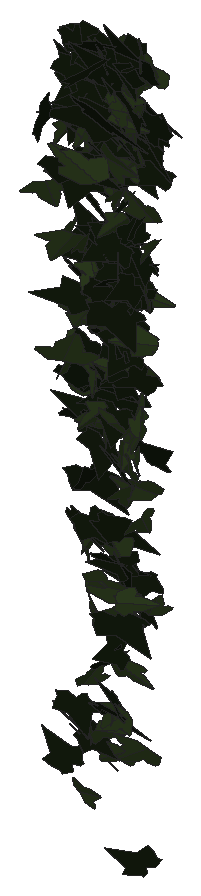
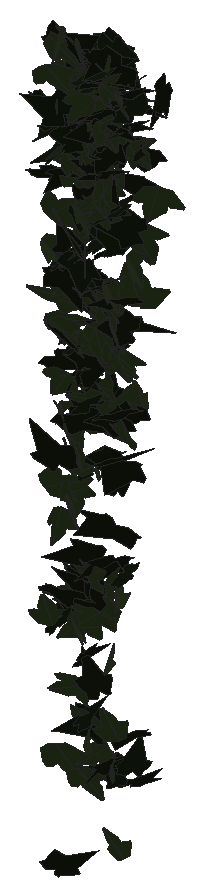
# SketchUp Ruby script. Lengths in millimetres.
U = 1.mm
M = Sketchup.active_model
def pt(a) = Geom::Point3d.new(a.map { |v| v * U })
def face(e, loops, mat)
  f = e.add_face(loops[0].map { |a| pt(a) })
  loops[1..].each { |l| e.add_face(l.map { |a| pt(a) }).erase! }
  f.material = f.back_material = mat if mat
  f
end
# faces: each face lists its corners as indices into pts; further lists are holes
def faces(e, pts, list, mat = nil) = list.each { |f| face(e, (f[0].is_a?(Array) ? f : [f]).map { |l| l.map { |i| pts[i] } }, mat) }
# xy, xz, yz: faces in a plane at the given z, y or x. An outline is a flat list of corners, or four numbers for a rectangle; further outlines are holes
def ring(l) = l.size == 4 ? [[l[0], l[1]], [l[2], l[1]], [l[2], l[3]], [l[0], l[3]]] : l.each_slice(2).to_a
def flat(e, list, mat, &to3) = list.each { |f| face(e, (f[0].is_a?(Array) ? f : [f]).map { |l| ring(l).map { |u, v| to3.(u, v) } }, mat) }
def xy(e, z, list, mat = nil) = flat(e, list, mat) { |x, y| [x, y, z] }
def xz(e, y, list, mat = nil) = flat(e, list, mat) { |x, z| [x, y, z] }
def yz(e, x, list, mat = nil) = flat(e, list, mat) { |y, z| [x, y, z] }
def lines(e, pts, list) = list.each { |a, b| e.add_line(pt(pts[a]), pt(pts[b])) }
# prism: a flat outline (further loops are holes) pulled along v
def prism(e, loops, v, mat = nil)
  f = face(e, loops, mat); d = Geom::Vector3d.new(v.map { |x| x * U })
  f.pushpull(f.normal.samedirection?(d) ? d.length : -d.length)
end
def box(e, o, s, mat = nil) = prism(e, [[o, [o[0] + s[0], o[1], o[2]], [o[0] + s[0], o[1] + s[1], o[2]], [o[0], o[1] + s[1], o[2]]]], [0, 0, s[2]], mat)
def at(x, y, z, deg = 0) = Geom::Transformation.translation(pt([x, y, z])) * Geom::Transformation.rotation(ORIGIN, Z_AXIS, deg.degrees)
def axes(o, x, y, z) = Geom::Transformation.new([*x, 0, *y, 0, *z, 0, *pt(o).to_a, 1])
def part(name) = M.definitions.add(name)
# library, detail: a bought-in or finely detailed component or shape, given as its bounding box
def library(name, o, s) = part(name).tap { |d| box(d.entities, o, s) }
def detail(e, o, s) = box(e.add_group.entities, o, s)
def put(e, d, t, mat = nil) = e.add_instance(d, t).tap { |i| i.material = mat if mat }
def group(e, t, mat = nil) = e.add_group.tap { |g| g.transformation = t; g.material = mat if mat }.entities
root = M.entities
M.materials.add("efeu1").color = [18, 25, 13]
M.materials.add("efeu2").color = [43, 57, 29]
c1 = part("ivyleaf_10")
p = [[0,12.8,-0.8],[-1.5,51.3,-10.9],[-4.9,51,-11.6],[-13.6,26.5,-7.3],[-13.2,15.9,-4.6],[-21.1,19.3,-7.2],
  [-29.5,16.3,-8.3],[-29.2,8.3,-6.2],[-19.7,-9.8,0.5],[-7.6,-13,4],[1,-12.2,5.8],[-0.4,51.1,-11.1],
  [-1.5,51.1,-10.9],[1,-12.4,5.9],[16.9,-12.4,3.5],[35.1,9.1,-5.1],[35,12.9,-6.1],[20.5,16.4,-4.9],
  [15.8,15,-3.8],[15.3,27.6,-7.1],[12.8,31.3,-7.8]]
faces(c1.entities,p,[[0,1,2,3,4,5,6,7,8,9,10],[11,12,0,13,14,15,16,17,18,19,20]],"efeu2")
c2 = part("ivyleaf_9")
p = [[39.1,54.8,31.7],[34.5,51.8,30.2],[-5.3,25.2,17.3],[-17.9,28.3,20.9],[-21.6,21.7,17],[-20.2,4.3,5.3],
  [-22.9,-0.3,2.5],[-17.1,-4,-0.6],[-2,-2.1,-1.2],[-0.7,-15.4,-10.1],[16.6,-22.3,-16.7],[21.1,-15.1,-12.5],
  [32.7,-10.7,-11],[46.1,-1.8,-6.6],[30.8,11.2,3.8]]
faces(c2.entities,p,[[0,1,2,3,4,5,6,7,8,9,10,11,12,13,14]],"efeu1")
put(root,c1,axes([2195.9,788.1,1105.5],[-1.48445,-0.69849,0.07567],[0.11289,0.04719,1.04701],[-1.33236,0.78222,0.0044]))
put(root,c2,axes([2211,826.6,1556.8],[1.10153,-0.62248,0.69314],[1.02059,-0.44467,-0.84712],[1.44988,0.78593,0.06969]))
put(root,c2,axes([2123.9,807.7,1529],[0.06736,0.10523,-1.08229],[-1.41364,0.79321,0.05283],[1.51148,0.73717,0.09764]))
put(root,c1,axes([2185.9,856.2,1418],[1.19765,0.4348,0.68302],[-1.13614,-0.33525,0.76342],[1.04104,-0.86609,0.04739]))
put(root,c1,axes([2141.6,863.4,1278.1],[-1.02412,-0.78375,0.34572],[-0.34417,-0.29513,-0.95054],[1.59356,-0.56743,0.01689]))
put(root,c2,axes([2137.7,850.3,1431],[0.19156,-0.13279,-0.94088],[0.74162,0.86869,-0.08091],[1.64937,-0.37518,0.14566]))
put(root,c1,axes([2096.4,861.2,1363.7],[-1.10138,-0.66826,-0.24815],[0.35472,0.16666,-0.88348],[1.3095,-0.6072,0.03061]))
put(root,c2,axes([2205.7,874.1,1520.3],[-0.43622,-0.2432,-0.87783],[-1.10818,-0.65698,0.33405],[-1.33317,0.62569,0.00955]))
put(root,c1,axes([2177.7,862.1,1294.8],[0.06368,-0.86339,-0.31702],[-0.02205,0.31681,-0.86404],[1.75033,0.0354,0.00065]))
put(root,c1,axes([2219.1,876.1,1443.2],[-0.62925,0.05857,0.92811],[1.62835,-0.36682,0.32794],[0.69353,0.91441,0.07211]))
put(root,c2,axes([2186.4,860.3,1609.5],[-0.55886,1.0553,-0.04247],[0.01541,-0.04183,-1.09538],[-2.01001,-0.29373,0.00341]))
put(root,c1,axes([2224.3,884.2,1046.1],[0.3322,0.31577,0.68802],[-0.61682,-0.60692,0.36077],[1.30205,-0.36808,-0.00463]))
put(root,c2,axes([2250.1,894.2,1212.7],[0.10304,-0.31171,-0.71457],[0.51528,-0.66419,0.31024],[-1.39137,-0.26906,0.06198]))
put(root,c2,axes([2145.1,887.9,1391.4],[-1.14627,-0.52715,-0.17902],[0.28365,0.10144,-0.80011],[1.02087,-0.62009,0.0213]))
put(root,c1,axes([2168.1,896.1,1022.4],[-0.02447,-0.49305,0.76391],[0.83949,-0.67144,-0.42595],[1.51314,0.36454,0.24867]))
put(root,c2,axes([2154.9,891,809.6],[0.46226,0.34244,0.63851],[-0.66837,-0.5334,0.41966],[1.20614,-0.42682,-0.01217]))
put(root,c1,axes([2156.9,886.7,1488.2],[1.00047,-0.78921,-0.03559],[-0.02329,0.03461,-0.94822],[1.50338,0.52575,0.00899]))
put(root,c2,axes([2126,885.9,269.5],[-0.87806,-0.60384,0.18477],[0.21995,0.14422,0.75991],[-1.18153,0.4756,0.00415]))
put(root,c1,axes([2175.6,902.7,944.1],[-0.0718,-0.35118,0.79561],[0.07092,-0.79628,-0.34971],[1.65364,0.0189,0.04954]))
put(root,c2,axes([2215.2,887.8,1156.4],[-0.43523,-0.69251,-0.56329],[0.26489,0.54671,-0.72863],[1.67817,-0.2659,-0.03108]))
put(root,c2,axes([2228.3,886.4,1056],[-1.19192,0.30407,0.34465],[-0.59238,0.14801,-0.69618],[-0.64361,-0.69935,0.00251]))
put(root,c2,axes([2156.4,902.8,1065.9],[0.03931,-0.79307,0.43311],[0.20855,-0.42782,-0.78862],[1.70709,0.07053,0.08637]))
put(root,c2,axes([2179.1,901,1534.1],[-1.08016,-0.19683,0.57563],[-0.89034,-0.36205,-0.58505],[0.74017,-0.72276,0.1363]))
put(root,c2,axes([2219.2,891.9,572],[-0.31181,-0.49695,-0.6787],[0.6745,0.58631,-0.51485],[1.45191,-0.3791,0.09342]))
put(root,c1,axes([2138.7,898.7,1526],[0.53915,-0.82773,0.04286],[0.02248,-0.04126,-0.87487],[1.57729,0.28352,-0.00218]))
put(root,c2,axes([2204.2,914.6,1266.8],[-0.86508,-0.53355,0.66094],[-0.61605,-0.58426,-0.69425],[1.49464,-0.54963,0.09639]))
put(root,c2,axes([2223.5,913.8,1081.3],[-0.60374,-0.76634,0.45104],[-0.32235,-0.41804,-0.8294],[1.66139,-0.35959,0.00298]))
put(root,c1,axes([2200.1,898.7,933.3],[-0.78514,-0.12179,0.76212],[-1.40688,-0.18605,-0.42987],[0.42222,-0.84641,-0.01517]))
put(root,c1,axes([2105.2,908.8,1463],[-0.09799,-0.67931,0.45198],[0.02847,-0.45359,-0.68002],[1.55263,-0.03456,0.04099]))
put(root,c1,axes([2096.4,903.2,991.3],[0.02775,-0.75101,-0.08197],[0.00604,-0.08192,0.75115],[-1.4378,-0.01484,0.00157]))
put(root,c2,axes([2118.8,914.6,1446.9],[0.14478,-0.58224,0.6331],[0.74638,-0.54218,-0.54575],[1.45694,0.33562,0.21667]))
put(root,c2,axes([2180.4,916.8,1259.8],[0.4557,-0.8888,-0.18002],[0.1809,-0.16057,0.91918],[-1.7164,-0.2529,0.04908]))
put(root,c2,axes([2174.1,912.2,1173.6],[-1.017,-0.0974,-0.54403],[1.051,-0.12473,-0.52008],[-0.04258,-0.7523,0.15667]))
put(root,c1,axes([2263.3,915.9,1095.7],[-0.09745,0.14739,0.80501],[-0.75629,-0.70959,0.10465],[1.36162,-0.38358,0.11574]))
put(root,c2,axes([2128.4,913.3,1135.9],[-0.91321,-0.05752,0.58833],[-1.08585,-0.15321,-0.4803],[0.29438,-0.74357,0.05346]))
put(root,c2,axes([2214.1,905.8,1581.1],[0.27263,-0.09433,0.92606],[-1.60092,0.38814,0.16965],[-0.75868,-0.85291,-0.02521]))
put(root,c2,axes([2117.7,910.7,374.3],[-0.22709,-0.75762,-0.22579],[0.04899,0.22451,-0.76691],[1.50378,-0.12173,-0.00912]))
put(root,c2,axes([2199.7,916,945.9],[-0.65144,-0.72229,-0.01541],[0.00749,0.01519,-0.79928],[1.37496,-0.3423,-0.00295]))
put(root,c1,axes([2213.7,918.2,1516],[-0.62352,0.44575,0.65062],[0.25239,-0.66336,0.52125],[1.47963,0.301,0.18526]))
put(root,c1,axes([2217.9,914.1,884.5],[0.07784,0.59628,-0.475],[-0.06334,-0.47383,-0.59769],[-1.44952,0.05273,0.00061]))
put(root,c1,axes([2176.6,898,1499.3],[-0.26285,-0.08684,-0.97194],[1.73927,0.33267,-0.15958],[0.65116,-0.92362,0.03391]))
put(root,c2,axes([2204.3,923.8,490],[-0.38277,-0.32158,0.7086],[-0.72085,-0.59888,-0.37929],[1.29372,-0.42884,-0.00168]))
put(root,c2,axes([2254.6,920.5,1032],[-0.06796,-0.07267,-0.76744],[-0.25126,-0.75633,0.07776],[-1.44544,0.13489,0.02257]))
put(root,c2,axes([2115.3,920.3,1569.2],[-0.42556,-0.8336,0.01086],[-0.00358,-0.01074,-0.86307],[1.58664,-0.22361,0.00097]))
put(root,c2,axes([2163.4,924.6,869.5],[-0.33078,-0.80386,0.29707],[-0.10038,-0.29251,-0.82238],[1.62795,-0.18137,0.00965]))
put(root,c1,axes([2190.8,925.7,1524.4],[-0.09339,-0.27072,0.80584],[0.25758,-0.79938,-0.26031],[1.59728,0.11308,0.08909]))
put(root,c1,axes([2211.1,909.7,377.9],[1.28908,-0.3914,-0.31063],[-0.50875,0.15825,-0.78227],[0.80348,0.72816,0.00304]))
put(root,c2,axes([2097.2,923.3,323],[1.0542,-0.54398,-0.11808],[0.16339,-0.08111,0.77635],[-1.04673,-0.56052,0.00226]))
put(root,c2,axes([2202.4,929.2,1002.6],[-0.39901,-0.53927,0.62119],[0.03972,-0.64433,-0.55231],[1.56509,-0.12113,0.17239]))
put(root,c1,axes([2227.8,899.5,602],[0.05539,-0.18103,-0.81104],[1.1182,0.57838,-0.10802],[1.11844,-0.5693,0.14816]))
put(root,c2,axes([2212.7,917.2,831.9],[0.40598,-0.68005,0.27052],[-0.10902,0.2654,0.71235],[-1.38865,-0.21966,0.02316]))
put(root,c1,axes([2197.7,928.1,1301],[-0.13531,-0.45967,0.71018],[-0.07774,-0.70999,-0.46363],[1.60815,-0.073,0.03734]))
put(root,c1,axes([2099.9,920.7,1262.3],[0.29299,-0.87739,0.21557],[0.1418,-0.20561,-0.89003],[1.71366,0.16702,0.03679]))
put(root,c2,axes([2121.1,920.7,303.8],[0.8713,-0.56256,0.32268],[0.39826,-0.24572,-0.72527],[1.16827,0.50332,0.00658]))
put(root,c2,axes([2170.7,912.7,375.1],[1.48661,-0.2162,0.19855],[0.36799,-0.04571,-0.81045],[0.42035,0.80465,0.00731]))
put(root,c2,axes([2214.5,931.9,1529.8],[0.16095,-0.67732,0.57446],[0.07982,-0.57337,-0.68221],[1.6884,0.09167,-0.02251]))
put(root,c1,axes([2219.4,918.8,840.3],[-1.2876,0.37459,0.1769],[0.28684,-0.09297,0.77328],[0.73438,0.69308,0.00812]))
put(root,c2,axes([2190.9,930.8,1205.5],[0.08679,0.1184,0.86302],[-0.32339,-0.8464,0.1251],[1.62605,-0.17465,-0.02118]))
put(root,c2,axes([2196,928.2,1606.8],[0.3106,-0.83329,0.14888],[0.00631,-0.15099,-0.84874],[1.61102,0.16125,-0.02538]))
put(root,c1,axes([2132.7,931.5,310.5],[-0.14426,0.11365,0.83409],[0.91119,-0.68301,0.13657],[1.31776,0.48472,-0.00312]))
put(root,c2,axes([2157,916.9,1257.4],[-0.77968,-0.73337,0.39954],[0.36714,0.34989,0.84003],[-1.54646,0.45281,-0.00201]))
put(root,c2,axes([2213.7,923.7,1208.9],[-0.7542,-0.67108,-0.32278],[0.27271,0.29009,-0.77904],[1.39078,-0.4208,-0.02228]))
put(root,c2,axes([2203.1,909.1,1199],[0.39013,0.74337,-0.04594],[-0.02616,-0.04387,-0.77111],[-1.41723,0.20544,0.00158]))
put(root,c2,axes([2199,939.5,1080.6],[-0.2509,-0.58996,0.70305],[-0.19429,-0.69643,-0.60355],[1.73589,-0.16322,0.03407]))
put(root,c2,axes([2108.9,915,995.6],[0.27177,0.07843,-0.84206],[1.17925,0.57151,0.1583],[1.09544,-0.63469,0.03849]))
put(root,c2,axes([2227.5,934.6,1174.4],[-0.94115,-0.55629,0.24804],[-0.17369,-0.24822,-0.73863],[1.14611,-0.49442,0.09174]))
put(root,c2,axes([2100.1,938,1462],[-0.26032,-0.67304,0.51776],[-0.22552,-0.50418,-0.68668],[1.60029,-0.18054,-0.01255]))
put(root,c1,axes([2236.7,921.7,905.6],[0.583,-0.69715,-0.10742],[-0.08403,0.09793,-0.76148],[1.33984,0.30949,-0.00102]))
put(root,c1,axes([2250.4,909.8,929.1],[0.06389,0.59128,-0.48542],[0.09105,0.48331,0.59202],[1.45311,-0.05628,-0.01575]))
put(root,c2,axes([2154.5,933.4,1587.2],[-0.36918,-0.84548,0.06048],[-0.02565,-0.05896,-0.86745],[1.61303,-0.19444,0.00005]))
put(root,c2,axes([2202.7,926.2,373.8],[0.2316,-0.79302,0.30633],[-0.00422,0.30916,0.80122],[-1.61797,-0.11432,0.04176]))
put(root,c2,axes([2244.9,918.4,1601.7],[0.51759,-0.40945,0.87162],[-0.91113,0.72838,0.49153],[-1.59027,-0.55058,0.00207]))
put(root,c1,axes([2208.3,937,914.9],[-0.08746,0.19222,0.7632],[0.25314,-0.75161,0.19731],[1.47635,0.14026,0.01138]))
put(root,c2,axes([2213.2,937.4,1230.6],[0.17494,-0.89699,-0.19736],[0.04999,-0.1957,0.90167],[-1.74727,-0.09541,0.00604]))
put(root,c2,axes([2145.1,936.4,1008.3],[0.29217,-0.58562,0.55405],[0.40726,-0.51418,-0.60276],[1.47928,0.25722,0.05652]))
put(root,c2,axes([2244.5,933.3,92.6],[0.03967,0.03805,0.771],[-1.35014,-0.30316,0.03414],[0.57926,-0.70921,0.02677]))
put(root,c2,axes([2238.3,917.9,1631.2],[-1.03703,0.55651,0.3232],[-0.41727,0.23763,-0.7788],[-1.15154,-0.58728,-0.00886]))
put(root,c1,axes([2141.9,938.1,1601.4],[-0.04561,-0.19022,0.85154],[1.19657,-0.59443,-0.11509],[1.15143,0.6102,0.15333]))
put(root,c2,axes([2202.7,939.4,1028.8],[-0.80466,-0.51969,0.3609],[-0.36028,-0.31028,-0.66856],[1.14903,-0.46123,0.04311]))
put(root,c2,axes([2154.6,940.9,1581.5],[-0.09187,-0.74776,0.44056],[0.13287,-0.44315,-0.74452],[1.64642,-0.00596,0.08467]))
put(root,c2,axes([2163.5,927.9,450.6],[0.76124,0.59419,0.45948],[-0.48725,-0.38155,0.71627],[1.34394,-0.4749,-0.00057]))
put(root,c1,axes([2190.5,921.9,1534],[1.22,0.38188,0.45288],[0.74645,0.2265,-0.74614],[-0.84496,0.75147,-0.00526]))
put(root,c2,axes([2109.3,942.2,1514.6],[-0.79742,-0.53929,0.51799],[-0.55442,-0.42913,-0.68241],[1.3107,-0.50962,0.02648]))
put(root,c1,axes([2245.9,913,862.2],[-0.05304,0.11799,0.75725],[-1.00158,0.54791,-0.10474],[-1.06035,-0.52345,0.06105]))
put(root,c2,axes([2194.7,937.6,622.2],[-0.25182,0.06257,0.84388],[0.18503,-0.84735,0.07807],[1.59981,0.10785,0.1238]))
put(root,c2,axes([2140.3,919.4,317.1],[0.30929,-0.46561,-0.62034],[-0.23652,0.60999,-0.4904],[1.45713,0.19784,0.05207]))
put(root,c1,axes([2214.6,934.8,1516.7],[0.03915,-0.74127,0.36329],[0.47335,-0.34095,-0.70977],[1.4981,0.1271,0.21477]))
put(root,c1,axes([2220.9,924.3,802.9],[-0.44617,-0.86981,-0.17617],[0.0504,0.17527,-0.90063],[1.68828,-0.2351,-0.01967]))
put(root,c1,axes([2234.2,927.1,1580],[-0.84692,-0.70945,-0.04313],[0.04106,0.03738,-0.83747],[1.3521,-0.44552,-0.00159]))
put(root,c1,axes([2251.2,935.8,803.1],[-0.7666,-0.0512,-0.76261],[-1.3268,-0.32881,0.39029],[-0.5964,0.79731,0.11198]))
put(root,c1,axes([2164.3,916.4,330.4],[-0.34279,-0.28273,-0.72286],[0.73287,0.61176,-0.33523],[1.28262,-0.42511,-0.00165]))
put(root,c2,axes([2160.8,940.5,1521.2],[0.30352,-0.75012,0.28949],[0.14659,-0.27952,-0.76671],[1.52321,0.17637,0.0161]))
put(root,c1,axes([2245.6,923.5,1093.2],[0.47949,-0.13166,-0.83357],[-1.32602,0.45841,-0.28299],[0.90626,0.74039,0.02697]))
put(root,c2,axes([2152.9,937,1473.3],[0.84058,-0.6628,0.18007],[0.18988,-0.14991,-0.79647],[1.2933,0.4528,-0.0001]))
put(root,c2,axes([2131.5,917.4,1615.8],[1.39129,0.45301,0.21296],[0.31969,0.13306,-0.85968],[-0.89744,0.74969,0.0239]))
put(root,c1,axes([2204.6,938.3,1404.8],[-0.80837,-0.67976,0.39362],[-0.29235,-0.36696,-0.79947],[1.46609,-0.44798,0.05761]))
put(root,c1,axes([2147.4,927.2,594.7],[-0.28478,-0.09225,0.88799],[1.56238,0.33964,0.17361],[-0.66778,0.834,0.02751]))
put(root,c2,axes([2147.4,936.3,1501.2],[-0.32724,-0.7198,-0.35832],[0.36149,0.31969,-0.73334],[1.48697,-0.23612,0.09942]))
put(root,c1,axes([2132.4,946,1175],[-0.66283,-0.45388,0.61207],[0.237,-0.69782,-0.44662],[1.43073,-0.09469,0.35754]))
put(root,c1,axes([2196.4,924.4,563.9],[-0.89821,-0.41579,-0.57038],[0.85732,0.35082,-0.62846],[1.03423,-0.65192,0.02559]))
put(root,c1,axes([2180.4,935.9,1405],[1.56511,0.1954,-0.41509],[-0.77574,-0.07991,-0.84513],[-0.40079,0.91771,0.01479]))
put(root,c1,axes([2256.8,927.3,1617.7],[-0.52392,0.1691,0.78607],[-1.48596,0.14226,-0.30403],[-0.36556,-0.82064,0.10927]))
put(root,c2,axes([2194.3,948.8,1024.5],[0.14324,-0.24162,-0.73314],[0.71159,-0.63303,0.24701],[-1.2853,-0.3774,0.05505]))
put(root,c1,axes([2244.4,923.5,1637.6],[0.49444,-0.61321,-0.55853],[0.22197,0.60648,-0.61161],[1.56293,0.10786,0.26356]))
put(root,c1,axes([2237.1,940.4,1191.3],[-0.32039,0.66822,-0.51384],[0.26263,-0.49507,-0.68902],[-1.58265,-0.21743,-0.01032]))
put(root,c2,axes([2202.2,936.8,1333.5],[-0.84551,0.58846,-0.47549],[0.52468,-0.38758,-0.73724],[-1.34089,-0.52272,0.01135]))
put(root,c1,axes([2127.1,942.9,1025.1],[0.33651,-0.2807,0.67421],[1.13048,-0.3483,-0.30079],[0.80864,0.60374,0.13994]))
put(root,c1,axes([2130.1,923.2,1417.1],[0.03956,-0.59617,-0.63833],[0.43013,0.62044,-0.5721],[1.60571,-0.15151,0.16898]))
put(root,c1,axes([2161.7,931.6,594],[-1.19787,-0.14357,-0.40165],[0.76865,0.02971,-0.6435],[0.26114,-0.74605,0.05167]))
put(root,c1,axes([2196.8,936.6,1628.6],[0.67355,-0.81168,-0.04704],[-0.03107,0.0442,-0.88547],[1.54707,0.35427,0.0027]))
put(root,c2,axes([2214.6,932.3,652.4],[-1.15033,0.37288,0.29163],[-0.47039,0.1548,-0.71018],[-0.76838,-0.653,-0.00182]))
put(root,c1,axes([2240,934.5,310],[-1.302,-0.16117,0.54079],[-1.00679,-0.11269,-0.70278],[0.37386,-0.86473,-0.00921]))
put(root,c1,axes([2170,950.1,359.1],[-0.11952,0.07664,0.88256],[0.85739,-0.75907,0.09797],[1.45173,0.45462,0.0148]))
put(root,c1,axes([2231.3,940,1519],[0.04416,-0.81164,0.15371],[0.20545,-0.14947,-0.80556],[1.55868,0.0427,0.10183]))
put(root,c2,axes([2177.2,928.5,1069.5],[1.30018,0.08931,-0.52708],[-1.00316,-0.03019,-0.68829],[-0.16978,0.86232,0.03049]))
put(root,c1,axes([2213.8,937.3,901.8],[0.75818,-0.81768,-0.10342],[-0.07095,0.09687,-0.90952],[1.567,0.40002,0.00886]))
put(root,c1,axes([2185.9,933.4,1096.5],[0.92099,-0.11141,-0.56654],[-0.97139,0.26307,-0.48769],[0.51379,0.69709,0.0935]))
put(root,c1,axes([2151.7,938.8,1165.5],[1.26054,-0.35838,-0.04558],[-0.07843,0.01961,-0.75306],[0.68307,0.6636,-0.00236]))
put(root,c2,axes([2241.8,940.8,1095],[-1.44674,0.22241,-0.20945],[0.38184,-0.06015,-0.79203],[-0.4385,-0.78619,0.00135]))
put(root,c1,axes([2146.3,950.9,875.9],[-0.07589,-0.04323,0.82819],[0.93156,-0.67056,-0.01144],[1.27414,0.48769,0.05769]))
put(root,c1,axes([2120.4,952.9,670.5],[-0.00686,-0.27996,0.77289],[0.48681,-0.73491,-0.26501],[1.48682,0.23933,0.09033]))
put(root,c1,axes([2156.9,946.8,1463.6],[-0.71767,-0.58511,0.42867],[-0.13191,-0.45186,-0.67774],[1.37415,-0.34896,0.15882]))
put(root,c1,axes([2190.9,938.1,286.8],[-1.03678,-0.1323,0.46695],[-0.86396,-0.10941,-0.56059],[0.32674,-0.70911,-0.00062]))
put(root,c2,axes([2246.7,930,1170.3],[-0.7195,0.45583,0.49738],[-0.57934,0.39357,-0.59206],[-1.14589,-0.4852,-0.01297]))
put(root,c2,axes([2073.5,951.2,1561.5],[0.32019,-0.68104,0.48598],[0.48288,-0.43084,-0.69159],[1.51734,0.28082,0.11754]))
put(root,c2,axes([2221.5,954.2,1234.2],[-0.0684,-0.71087,0.4263],[0.0144,-0.42697,-0.71134],[1.57748,-0.02692,0.02498]))
put(root,c2,axes([2122,941.6,1544.3],[0.08659,-0.81472,-0.45597],[0.00094,0.45653,-0.81568],[1.7769,0.03946,0.02265]))
put(root,c2,axes([2152.7,940.3,634],[1.04884,0.18256,-0.49055],[0.87207,0.17604,0.58028],[0.48151,-0.71649,0.01758]))
put(root,c1,axes([2106.9,944.3,1569],[0.76958,-0.75752,0.05912],[0.05041,-0.05288,-0.85869],[1.44522,0.40523,-0.00153]))
put(root,c1,axes([2156.1,954.1,1135.5],[-0.45015,-0.29597,0.6492],[0.20957,-0.69089,-0.27485],[1.34162,0.00862,0.26076]))
put(root,c1,axes([2239.1,932.7,748.8],[-0.36215,-0.7711,-0.50217],[0.26058,0.48336,-0.7941],[1.73184,-0.23398,0.01447]))
put(root,c2,axes([2124.7,933,974.6],[0.15097,0.10384,-0.80539],[0.94702,0.63329,0.13066],[1.22137,-0.50388,-0.00176]))
put(root,c1,axes([2103.6,946.3,175.7],[-0.75218,0.09706,0.58681],[1.05089,-0.20199,0.4053],[0.42074,0.67804,0.03674]))
put(root,c1,axes([2112.8,942.6,1092.2],[-1.17193,-0.33553,0.25023],[-0.39845,-0.13854,-0.70096],[0.6898,-0.65007,0.02023]))
put(root,c2,axes([2272.4,930.5,1488.4],[-0.11861,0.12848,0.87859],[-0.83716,0.76062,-0.14243],[-1.46799,-0.44414,0.01023]))
put(root,c1,axes([2196.7,940.8,450.6],[-0.91837,0.06416,-0.54493],[1.02433,-0.08582,-0.4867],[-0.20315,-0.7228,0.00942]))
put(root,c1,axes([2137.8,938.8,1082.3],[-0.30334,0.05236,0.7381],[-1.40727,0.01748,-0.16091],[-0.05363,-0.75491,0.04747]))
put(root,c1,axes([2092.4,929.6,1033.7],[0.12899,-0.45707,-0.70584],[0.68139,0.65642,-0.39069],[1.4481,-0.26816,0.24671]))
put(root,c1,axes([2101.7,954.1,640.4],[-0.71196,0.23327,0.68753],[0.79815,-0.56192,0.41884],[1.12793,0.54487,0.1376]))
put(root,c1,axes([2189.9,952.5,573.7],[0.52515,-0.73905,0.40423],[0.34292,-0.36374,-0.78801],[1.5661,0.32747,0.037]))
put(root,c1,axes([2129.2,941.3,1175.3],[0.46637,-0.08512,-0.88949],[1.69563,-0.04729,0.24997],[-0.13011,-0.92142,0.06934]))
put(root,c2,axes([2195.8,956,960],[-0.12779,-0.08179,-0.85804],[-0.45948,-0.8244,0.09748],[-1.57476,0.24718,0.04119]))
put(root,c2,axes([2126,939.3,708.8],[0.30045,-0.60152,-0.6506],[0.00398,0.6611,-0.61071],[1.68634,0.10561,0.11735]))
put(root,c2,axes([2146.8,949.4,1358.5],[1.25802,-0.36637,0.42115],[-0.63748,0.26185,0.7535],[-0.84986,-0.73873,0.05822]))
put(root,c2,axes([2158,961.4,1598.7],[-0.5123,-0.64368,0.49469],[0.11144,-0.53521,-0.66454],[1.54101,-0.17528,0.21251]))
put(root,c2,axes([2229.5,952.4,860.4],[-0.3799,-0.0904,0.83266],[0.98214,-0.68748,0.04907],[1.25552,0.51043,0.21356]))
put(root,c1,axes([2186.3,946.5,1345.9],[-0.04161,-0.84255,0.00958],[0.00088,-0.00959,-0.84284],[1.60365,-0.02186,0.00071]))
put(root,c2,axes([2088.6,956.5,1319.6],[0.69682,-0.76582,0.44652],[0.37975,-0.39952,-0.84881],[1.64387,0.41691,0.00681]))
put(root,c2,axes([2087.4,946.4,1609.6],[0.48846,-0.75527,-0.28664],[0.0319,0.30567,-0.79041],[1.53714,0.23366,0.10749]))
put(root,c2,axes([2126.2,961.3,1500],[-0.54956,-0.61238,0.45857],[-0.01008,-0.48854,-0.65573],[1.45601,-0.23452,0.16855]))
put(root,c2,axes([2086.5,945.6,698.4],[0.87204,-0.61319,-0.18487],[-0.17178,0.16321,-0.76508],[1.20675,0.46635,0.02468]))
put(root,c2,axes([2222.8,962.2,564],[-0.107,-0.46218,0.69257],[-0.03507,-0.69328,-0.46416],[1.58426,-0.04656,0.0365]))
put(root,c1,axes([2182,944.7,1191.3],[-1.16583,0.1189,-0.4308],[0.80528,-0.08099,-0.624],[-0.27379,-0.74449,-0.00092]))
put(root,c1,axes([2095.5,943.5,945.9],[1.25686,-0.34254,0.078],[-0.10559,0.0623,0.74336],[-0.66022,-0.66206,0.0296]))
put(root,c2,axes([2236.3,958.5,1477.5],[0.13803,-0.82185,0.23649],[0.02628,-0.23619,-0.82502],[1.6274,0.07352,-0.00674]))
put(root,c2,axes([2205.5,955.8,1439],[-1.36237,-0.23108,0.31821],[-0.57684,-0.09693,-0.7522],[0.47692,-0.77735,-0.0008]))
put(root,c1,axes([2212.3,945,1166.1],[-0.10776,-0.14446,-0.8194],[1.58081,-0.05798,-0.04717],[-0.09287,-0.8193,0.14782]))
put(root,c2,axes([2132.4,939.4,1478.4],[1.30285,-0.01253,-0.44843],[-0.85174,0.03763,-0.68423],[0.05918,0.81749,0.02462]))
put(root,c2,axes([2150.1,939.7,706.5],[0.21483,-0.084,-0.88602],[1.03596,0.71312,0.00174],[1.34011,-0.5378,0.14069]))
put(root,c1,axes([2240,945.6,1318.6],[-1.2963,0.19262,-0.48357],[-0.88515,0.13242,0.70783],[0.44486,0.82476,-0.00071]))
put(root,c2,axes([2159.9,958.5,995.3],[0.42358,-0.64511,0.45029],[0.33336,-0.41559,-0.68196],[1.4597,0.28211,0.02508]))
put(root,c2,axes([2185.7,944,1209.7],[-0.76267,0.67454,-0.16754],[0.15127,-0.14765,-0.78456],[-1.31411,-0.40848,0.00692]))
put(root,c1,axes([2115.6,947.3,392.9],[-0.43181,-0.75915,0.11242],[0.11405,0.09935,0.79181],[-1.45611,0.2329,0.02868]))
put(root,c1,axes([2148,948.5,1109.1],[-1.14475,0.35762,-0.39824],[0.58203,-0.26203,-0.6972],[-0.83604,-0.6721,0.05992]))
put(root,c2,axes([2131.7,957.3,891.5],[-0.50802,-0.84508,-0.18534],[-0.09855,-0.17801,0.88623],[-1.64363,0.27188,0.00415]))
put(root,c2,axes([2131.6,953,1521.4],[-0.91469,-0.4786,-0.46938],[0.77759,0.24874,-0.67197],[1.01146,-0.62404,0.09213]))
put(root,c1,axes([2141.9,945.6,1003.1],[-0.47782,-0.13216,-0.68773],[1.33193,-0.02029,-0.25158],[0.04935,-0.73184,0.13117]))
put(root,c1,axes([2123.6,960.1,1596.4],[0.02176,-0.59414,0.59444],[0.28319,-0.58367,-0.58624],[1.57429,0.1132,0.09724]))
put(root,c2,axes([2148.1,964.2,1540.5],[-0.61022,-0.74132,0.36975],[-0.22423,-0.35165,-0.80718],[1.56062,-0.34039,0.0286]))
put(root,c1,axes([2124.3,936.6,1511],[-0.31502,-0.50699,-0.67074],[0.65728,0.58229,-0.52536],[1.45898,-0.3718,0.09185]))
put(root,c1,axes([2221.8,943.9,933.9],[0.89912,-0.64562,0.27146],[-0.31824,0.21399,0.79996],[-1.29438,-0.50108,-0.00812]))
put(root,c2,axes([2069.5,951.3,1343.4],[1.14118,-0.41124,0.45427],[0.70829,-0.26053,-0.72708],[0.92649,0.70571,-0.0037]))
put(root,c2,axes([2168.9,944.7,1428.1],[-0.0148,-0.50441,-0.69018],[0.53291,0.65063,-0.47866],[1.53722,-0.23041,0.1593]))
put(root,c1,axes([2144.3,951.7,1364.2],[1.53277,0.17384,-0.4092],[-0.75996,-0.08949,-0.82391],[-0.37207,0.89892,-0.00289]))
put(root,c1,axes([2242.1,957.4,1584],[-1.10836,-0.41135,0.43698],[-0.24778,-0.50781,-0.65153],[1.11497,-0.52176,0.2896]))
put(root,c2,axes([2198.2,946,1411.1],[-0.03356,-0.64084,-0.62366],[0.10275,0.62188,-0.64054],[1.69877,-0.05027,0.02642]))
put(root,c2,axes([2215.8,955.9,626.5],[-1.26228,-0.38951,-0.27534],[0.4518,0.1395,-0.76916],[0.78742,-0.70445,-0.00007]))
put(root,c2,axes([2080.8,954.6,1156.8],[1.01566,-0.51151,0.41089],[0.54367,-0.29567,-0.73909],[1.12413,0.60515,-0.0138]))
put(root,c1,axes([2179.3,943.4,666.7],[1.19564,-0.18605,0.63949],[-1.1648,0.18541,0.65519],[-0.49988,-0.87706,0.00285]))
put(root,c2,axes([2122.3,964,1606.1],[-1.32716,-0.48736,0.10601],[0.14193,-0.28207,-0.80617],[0.93856,-0.64649,0.27182]))
put(root,c1,axes([2136.5,947.2,1400],[-0.3318,-0.84804,-0.19718],[0.07346,0.19337,-0.86577],[1.65541,-0.17856,-0.0011]))
put(root,c1,axes([2147,954.4,1354.6],[1.13278,-0.25977,0.46688],[0.86534,-0.12079,-0.64684],[0.53403,0.74676,0.05778]))
put(root,c1,axes([2154.2,956.1,1381.8],[0.23101,0.66374,-0.44421],[-0.28861,-0.42198,-0.67197],[-1.49238,0.18435,0.06119]))
put(root,c2,axes([2130.4,962.3,1227.2],[-0.26557,-0.79423,0.16324],[-0.02785,-0.16315,-0.80628],[1.54292,-0.13965,0.01355]))
put(root,c2,axes([2103.4,940.3,898.4],[1.24227,0.46953,-0.12028],[-0.19308,-0.06494,-0.80403],[-0.90203,0.66053,0.00645]))
put(root,c1,axes([2206.4,951.1,788.4],[0.55176,-0.71346,-0.09655],[-0.06297,0.09078,-0.77011],[1.36879,0.29178,0.00349]))
put(root,c1,axes([2245.9,958.4,1260.9],[0.09425,-0.69104,0.33542],[-0.00577,-0.33629,-0.69239],[1.46193,0.04323,-0.02436]))
put(root,c2,axes([2104.4,957.4,1206.3],[-0.42313,-0.79633,-0.23959],[0.19873,0.21931,-0.82582],[1.57016,-0.24236,0.03995]))
put(root,c1,axes([2169.7,939,1542.2],[-0.7603,0.48953,0.5391],[-0.61851,0.43041,-0.63166],[-1.24024,-0.51475,-0.01547]))
put(root,c1,axes([2121.5,957.3,516.5],[-0.61177,0.53957,0.45116],[0.41441,-0.39533,0.62794],[1.27282,0.38805,0.0124]))
put(root,c1,axes([2121.8,954.2,1222.7],[0.05333,-0.80758,0.08612],[-0.01056,-0.08636,-0.80803],[1.54567,0.02727,-0.00849]))
put(root,c2,axes([2210.8,942.1,1265.5],[-0.46738,-0.30907,0.69732],[0.9906,0.46759,0.39055],[-1.06114,0.57264,0.05746]))
put(root,c2,axes([2190.1,950.3,1271.5],[-0.13171,0.67805,0.50529],[0.10351,-0.50236,0.68157],[1.60604,0.08798,-0.00249]))
put(root,c2,axes([2220.3,948,1211.6],[0.13094,0.67218,-0.35486],[-0.1028,-0.35108,-0.6755],[-1.44296,0.08601,0.01592]))
put(root,c2,axes([2137.3,963.4,1431.6],[-0.66493,-0.72606,0.10089],[-0.0329,-0.10357,-0.80522],[1.39473,-0.34859,0.0291]))
put(root,c1,axes([2196.8,948.6,1474.5],[1.08255,-0.53982,-0.22905],[-0.07638,0.28252,-0.7655],[1.11343,0.54423,0.17019]))
put(root,c1,axes([2151,950.8,1118.2],[-1.3146,-0.21362,0.19897],[-0.35897,-0.06354,-0.72299],[0.42406,-0.716,0.0048]))
put(root,c2,axes([2190.8,939.7,1239.6],[0.32683,0.74034,0.09604],[0.03811,0.09395,-0.75999],[-1.42031,0.17288,0.00171]))
put(root,c2,axes([2095.9,945.6,1380.7],[1.04238,-0.49041,-0.45193],[-0.37447,0.43995,-0.71585],[1.21272,0.55737,0.16741]))
put(root,c1,axes([2132.2,958.1,1516],[-0.25624,-0.76169,0.27538],[-0.10633,-0.26975,-0.77346],[1.5378,-0.14557,-0.0076]))
put(root,c2,axes([2214.9,961.6,1516.1],[0.75522,-0.53999,0.58577],[0.6662,-0.46969,-0.67011],[1.36207,0.52914,0.00297]))
put(root,c2,axes([2178.5,960,1479.7],[0.84848,-0.5495,0.46515],[0.58652,-0.3488,-0.70741],[1.23831,0.54172,0.01634]))
put(root,c2,axes([2104.1,963.9,998.1],[-0.55379,-0.73419,0.07749],[-0.02746,-0.07762,-0.78961],[1.40481,-0.29094,0.01511]))
put(root,c1,axes([2107.4,957.5,1153.5],[0.40537,-0.80801,0.14369],[0.10541,-0.13396,-0.83539],[1.55836,0.21925,0.01913]))
put(root,c1,axes([2244.4,955,565.8],[-0.67531,-0.63538,0.01556],[0.03255,0.00827,0.72766],[-1.20917,0.35507,0.0109]))
put(root,c1,axes([2165,948.1,1548.3],[-1.27,-0.33583,-0.36302],[0.61086,0.16974,-0.74701],[0.71604,-0.74045,-0.0066]))
put(root,c2,axes([2113.3,952.6,783.5],[-0.413,-0.29265,-0.81068],[1.19301,0.52017,-0.35557],[1.12581,-0.65857,0.0794]))
put(root,c2,axes([2149.7,936.8,1493.3],[0.51867,0.2953,0.71633],[0.91192,0.53251,-0.40181],[-1.15884,0.55121,0.00442]))
put(root,c2,axes([2248.6,965.4,1401.9],[-1.24797,-0.3778,0.30297],[-0.49596,-0.15458,-0.75676],[0.77686,-0.70559,0.00357]))
put(root,c1,axes([2195.2,963.8,1444.1],[-0.1641,-0.75373,0.44267],[0.09425,-0.44831,-0.7537],[1.66093,-0.04903,0.08651]))
put(root,c2,axes([2223.2,956,1445],[0.80067,-0.67566,-0.16153],[-0.16709,0.13561,-0.79592],[1.31154,0.42975,-0.00279]))
put(root,c1,axes([2218.4,952.2,1022.2],[-1.2621,0.26247,-0.12788],[0.21284,-0.06482,-0.71295],[-0.51329,-0.67225,0.01881]))
put(root,c1,axes([2216.5,956.2,1451.9],[0.14367,0.78451,-0.21886],[-0.01504,-0.21909,-0.78803],[-1.55002,0.07484,-0.01264]))
